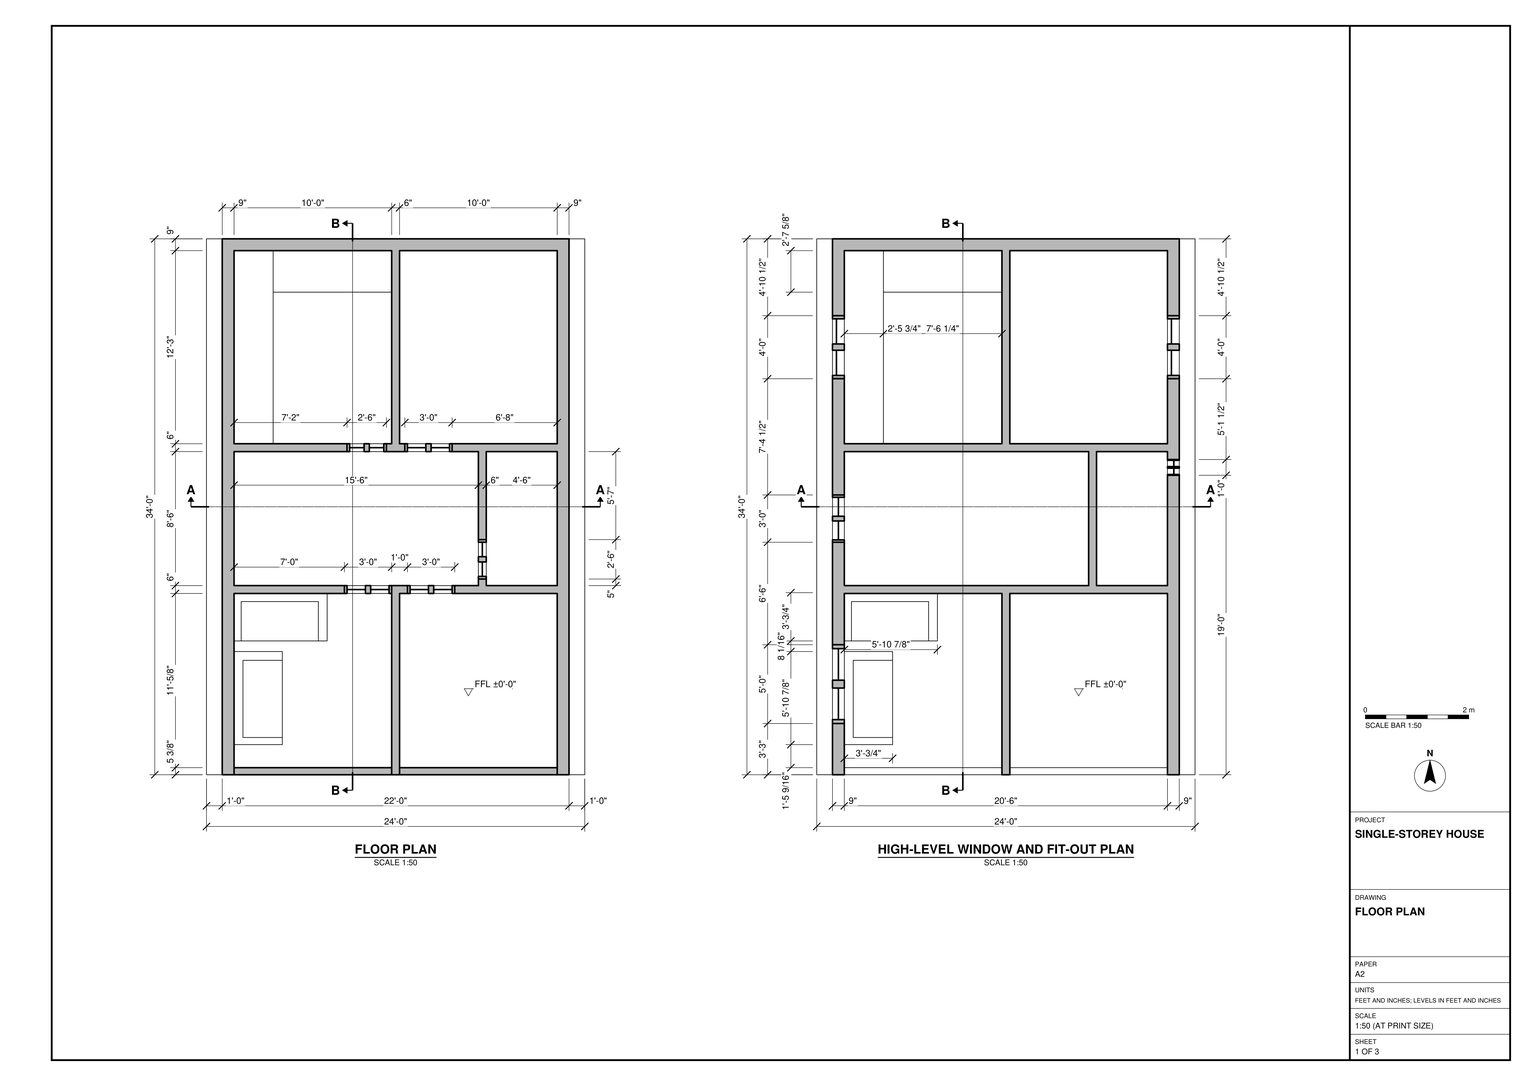
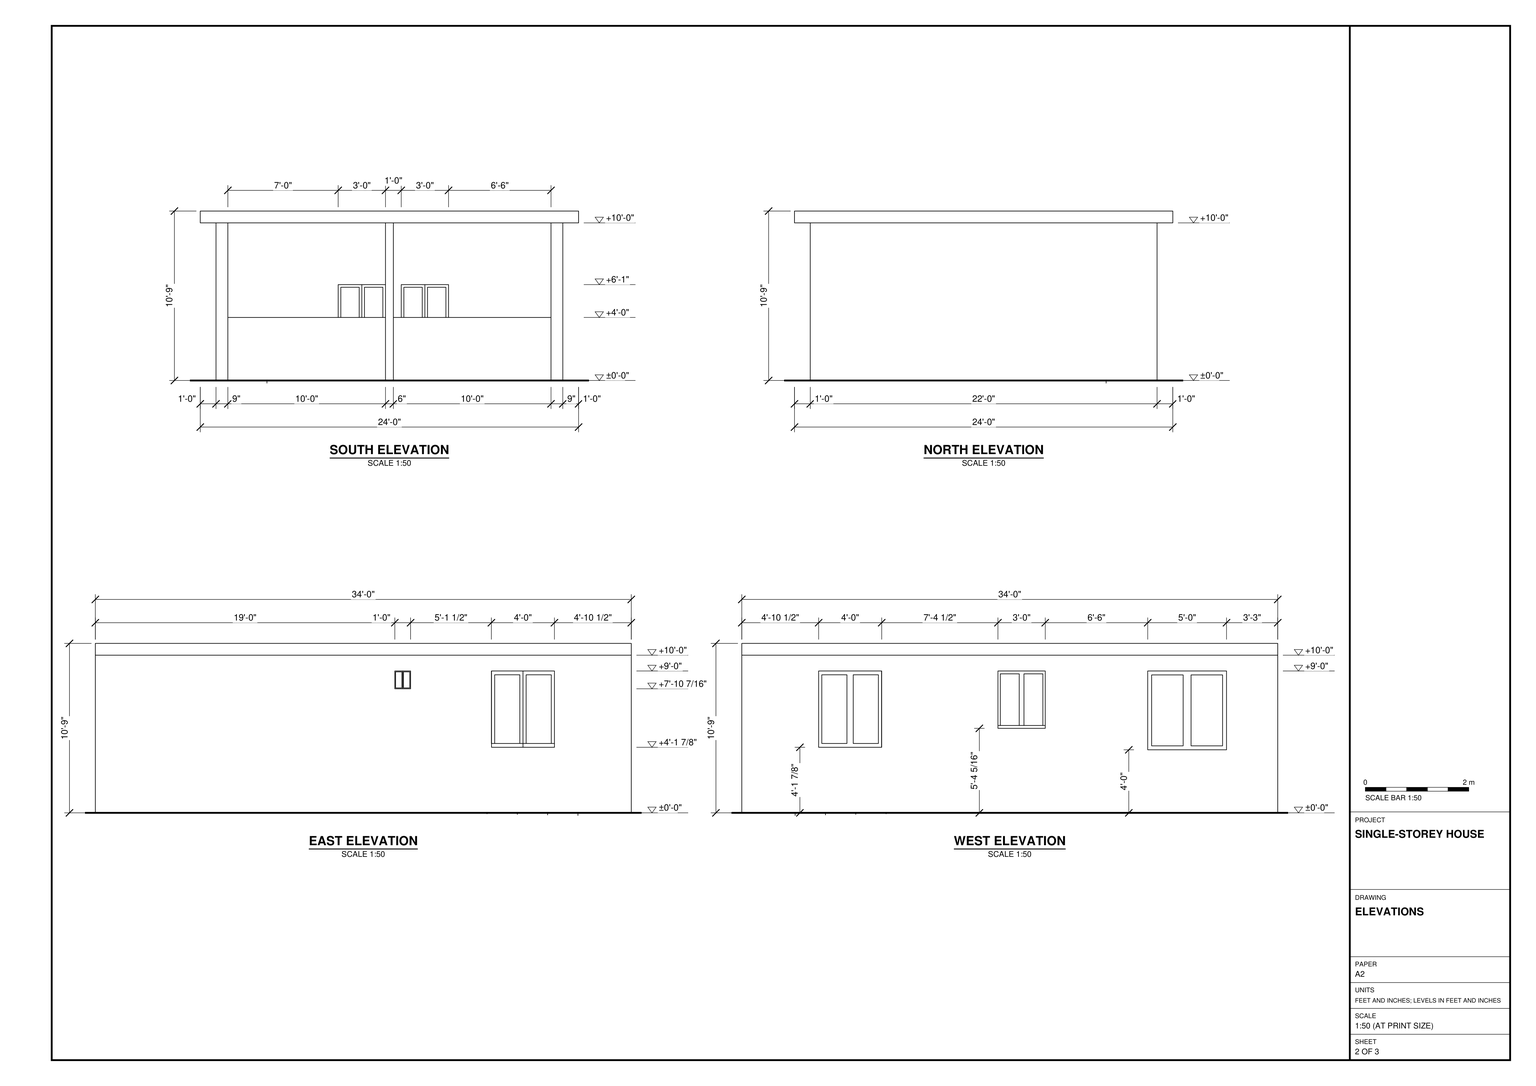
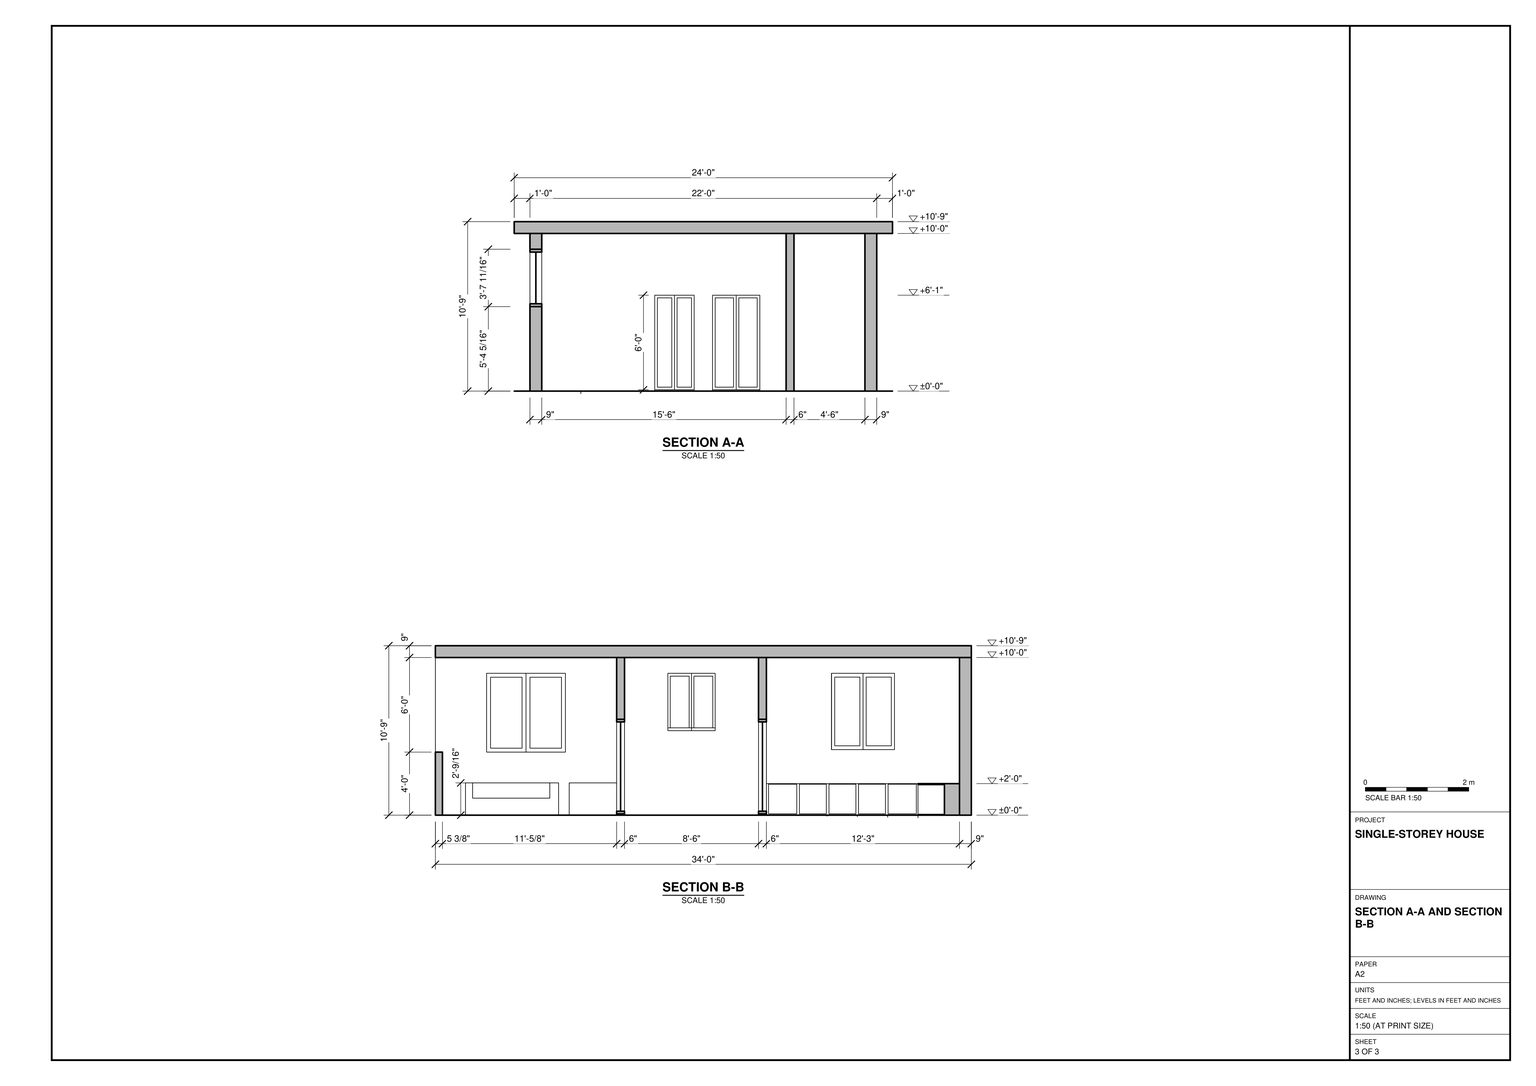
Build the single-storey house shown in task_files/diagram_01.pdf. Work in feet and inches. Set the finished floor at ±0'-0" and orient the plan with north at the top. The overall dimensions, including the roof, are 24'-0" east to west, 34'-0" north to south and 10'-9" high.

Model the floor, the 9" full-height exterior walls and the 6" interior partitions. Divide each end of the house into two equal-width rooms. In the middle band, place the wider room on the west and the narrow room on the east. Use the sections to distinguish the low south wall from the full-height walls behind it. Set the underside of the flat roof at +10'-0" and extend it 1'-0" beyond each side wall.

Use the floor plan to place the interior door units and the high-level plan to locate the exterior windows. Match the window widths and sill heights to the elevations rather than repeating one window size throughout. Model the low built-in joinery in the northwest room and the two low furniture pieces set at right angles in the southwest room. Any decor or loose items may be represented by suitable library components.

Keep the shell elements, including the walls, floor slab and roof, and each furniture or joinery piece in separate groups or components. Use components for repeated parts. Save one SketchUp model as output_files/single_storey_house_with_an_overhanging_flat_roof.skp.

# SketchUp Ruby script. Lengths in inches.
U = 1.inch
M = Sketchup.active_model
def pt(a) = Geom::Point3d.new(a.map { |v| v * U })
def face(e, loops, mat)
  f = e.add_face(loops[0].map { |a| pt(a) })
  loops[1..].each { |l| e.add_face(l.map { |a| pt(a) }).erase! }
  f.material = f.back_material = mat if mat
  f
end
# faces: each face lists its corners as indices into pts; further lists are holes
def faces(e, pts, list, mat = nil) = list.each { |f| face(e, (f[0].is_a?(Array) ? f : [f]).map { |l| l.map { |i| pts[i] } }, mat) }
# xy, xz, yz: faces in a plane at the given z, y or x. An outline is a flat list of corners, or four numbers for a rectangle; further outlines are holes
def ring(l) = l.size == 4 ? [[l[0], l[1]], [l[2], l[1]], [l[2], l[3]], [l[0], l[3]]] : l.each_slice(2).to_a
def flat(e, list, mat, &to3) = list.each { |f| face(e, (f[0].is_a?(Array) ? f : [f]).map { |l| ring(l).map { |u, v| to3.(u, v) } }, mat) }
def xy(e, z, list, mat = nil) = flat(e, list, mat) { |x, y| [x, y, z] }
def xz(e, y, list, mat = nil) = flat(e, list, mat) { |x, z| [x, y, z] }
def yz(e, x, list, mat = nil) = flat(e, list, mat) { |y, z| [x, y, z] }
def lines(e, pts, list) = list.each { |a, b| e.add_line(pt(pts[a]), pt(pts[b])) }
# prism: a flat outline (further loops are holes) pulled along v
def prism(e, loops, v, mat = nil)
  f = face(e, loops, mat); d = Geom::Vector3d.new(v.map { |x| x * U })
  f.pushpull(f.normal.samedirection?(d) ? d.length : -d.length)
end
def box(e, o, s, mat = nil) = prism(e, [[o, [o[0] + s[0], o[1], o[2]], [o[0] + s[0], o[1] + s[1], o[2]], [o[0], o[1] + s[1], o[2]]]], [0, 0, s[2]], mat)
def at(x, y, z, deg = 0) = Geom::Transformation.translation(pt([x, y, z])) * Geom::Transformation.rotation(ORIGIN, Z_AXIS, deg.degrees)
def axes(o, x, y, z) = Geom::Transformation.new([*x, 0, *y, 0, *z, 0, *pt(o).to_a, 1])
def part(name) = M.definitions.add(name)
# library, detail: a bought-in or finely detailed component or shape, given as its bounding box
def library(name, o, s) = part(name).tap { |d| box(d.entities, o, s) }
def detail(e, o, s) = box(e.add_group.entities, o, s)
def put(e, d, t, mat = nil) = e.add_instance(d, t).tap { |i| i.material = mat if mat }
def group(e, t, mat = nil) = e.add_group.tap { |g| g.transformation = t; g.material = mat if mat }.entities
root = M.entities
M.materials.add("[Carrera Marble]").color = [207, 207, 207]
M.materials.add("[Color M06]").color = [86, 86, 86]
M.materials.add("[Fencing Picket Concave]").color = [160, 160, 160]
M.materials.add("[Stone Brushed Khaki]").color = [226, 197, 133]
M.materials.add("[Translucent Glass Blue]").color = [100, 149, 237]
M.materials["[Translucent Glass Blue]"].alpha = 0.5
M.materials.add("[Wood Cherry Original]").color = [152, 86, 42]
M.materials.add("[Wood Floor]").color = [155, 105, 61]
M.materials.add("[Wood OSB]").color = [240, 195, 122]
c1 = part("Component\#1")
xy(c1.entities,0,[[0,0,36.75,70.875]],"[Carrera Marble]")
xy(c1.entities,12.9375,[[6.77,5.43,36.75,64.17]],"[Color M06]")
xy(c1.entities,24.5625,[[0,0,36.75,0,36.75,5.43,6.77,5.43,6.77,64.17,36.75,64.17,36.75,70.875,0,70.875]],"[Color M06]")
xz(c1.entities,0,[[0,0,36.75,24.5625]],"[Color M06]")
xz(c1.entities,5.43,[[6.77,12.9375,36.75,24.5625]],"[Color M06]")
xz(c1.entities,64.17,[[6.77,12.9375,36.75,24.5625]],"[Color M06]")
xz(c1.entities,70.875,[[0,0,36.75,24.5625]],"[Color M06]")
yz(c1.entities,0,[[0,0,70.875,24.5625]],"[Carrera Marble]")
yz(c1.entities,6.77,[[5.43,12.9375,64.17,24.5625]],"[Color M06]")
yz(c1.entities,36.75,[[0,0,70.875,0,70.875,24.5625,64.17,24.5625,64.17,12.9375,5.43,12.9375,5.43,24.5625,0,24.5625]],"[Color M06]")
c2 = part("Group\#2")
xy(c2.entities,0,[[0,0,9,30],[0,30,9,60]])
xy(c2.entities,3,[[0,3,4.5,27],[4.5,3,9,27],[0,33,4.5,57],[4.5,33,9,57]])
xy(c2.entities,57,[[0,3,4.5,27],[4.5,3,9,27],[0,33,4.5,57],[4.5,33,9,57]])
xy(c2.entities,60,[[0,0,9,30],[0,30,9,60]])
xz(c2.entities,0,[[0,0,9,60]])
xz(c2.entities,3,[[0,3,4.5,57],[4.5,3,9,57]])
xz(c2.entities,27,[[0,3,4.5,57],[4.5,3,9,57]])
xz(c2.entities,33,[[0,3,4.5,57],[4.5,3,9,57]])
xz(c2.entities,57,[[0,3,4.5,57],[4.5,3,9,57]])
xz(c2.entities,60,[[0,0,9,60]])
yz(c2.entities,0,[[[0,0,60,60],[3,3,27,57],[33,3,57,57]]])
yz(c2.entities,4.5,[[3,3,27,57],[33,3,57,57]],"[Translucent Glass Blue]")
yz(c2.entities,9,[[[0,0,30,60],[3,3,27,57]],[[30,0,60,60],[33,3,57,57]]])
c3 = part("Group\#5")
xy(c3.entities,0,[[0,0,36,6]],"[Carrera Marble]")
xy(c3.entities,1,[[0,0,36,6]],"[Stone Brushed Khaki]")
xz(c3.entities,0,[[0,0,36,1]],"[Stone Brushed Khaki]")
xz(c3.entities,6,[[0,0,36,1]],"[Stone Brushed Khaki]")
yz(c3.entities,0,[[0,0,6,1]],"[Carrera Marble]")
yz(c3.entities,36,[[0,0,6,1]],"[Carrera Marble]")
c4 = part("Group\#3")
xy(c4.entities,0,[[0,0,30,6]])
xy(c4.entities,1,[[0,0,30,6]],"[Wood OSB]")
xz(c4.entities,0,[[0,0,30,1]],"[Wood OSB]")
xz(c4.entities,6,[[0,0,30,1]],"[Wood OSB]")
yz(c4.entities,0,[[0,0,6,1]])
yz(c4.entities,30,[[0,0,6,1]])
c5 = part("Group\#9")
xy(c5.entities,0,[[0,-6,15,0],[15,-6,30,0]])
xy(c5.entities,2,[[2,-6,13,-3],[17,-6,28,-3],[2,-3,13,0],[17,-3,28,0]])
xy(c5.entities,70,[[2,-6,13,-3],[17,-6,28,-3],[2,-3,13,0],[17,-3,28,0]])
xy(c5.entities,72,[[0,-6,30,0]])
xz(c5.entities,-6,[[[0,0,15,72],[2,2,13,70]],[[15,0,30,72],[17,2,28,70]]])
xz(c5.entities,-3,[[2,2,13,70],[17,2,28,70]])
xz(c5.entities,0,[[[0,0,30,72],[17,2,28,70],[2,2,13,70]]])
yz(c5.entities,0,[[-6,0,0,72]])
yz(c5.entities,2,[[-6,2,-3,70],[-3,2,0,70]])
yz(c5.entities,13,[[-6,2,-3,70],[-3,2,0,70]])
yz(c5.entities,17,[[-6,2,-3,70],[-3,2,0,70]])
yz(c5.entities,28,[[-6,2,-3,70],[-3,2,0,70]])
yz(c5.entities,30,[[-6,0,0,72]])
c6 = part("Group\#11")
xy(c6.entities,0,[[0,0,120,5.39]],"[Carrera Marble]")
xy(c6.entities,48,[[0,0,120,5.39]],"[Carrera Marble]")
xz(c6.entities,0,[[0,0,120,48]],"[Fencing Picket Concave]")
xz(c6.entities,5.39,[[0,0,120,48]],"[Carrera Marble]")
yz(c6.entities,0,[[0,0,5.39,48]],"[Carrera Marble]")
yz(c6.entities,120,[[0,0,5.39,48]],"[Carrera Marble]")
xy(root,0,[[0,0,12,408],[12,0,21,0,21,138,105,138,105,144,21,144,21,246,107,246,107,252,21,252,21,399,141,399,141,252,137,252,137,246,151,246,151,252,147,252,147,399,267,399,267,252,187,252,187,246,207,246,207,179,213,179,213,246,267,246,267,144,213,144,213,149,207,149,207,144,189,144,189,138,267,138,267,0,276,0,276,408,12,408],[276,0,288,408],[107,246,137,252]])
xy(root,0,[[147,0,267,0,267,138,189,138,189,144,207,144,207,149,213,149,213,144,267,144,267,246,213,246,213,179,207,179,207,246,21,246,21,144,153,144,153,138,147,138],[21,5.39,141,138],[50.76,252,141,367.4],[147,252,267,399]],"[Carrera Marble]")
xy(root,48,[[12,39,21,99]])
xy(root,49.9,[[12,301.5,21,349.5]])
xy(root,52.81,[[267,301.5,276,349.5]])
xy(root,66.5,[[12,177,21,213]])
xy(root,73,[[105,138,141,144],[153,138,189,144],[207,149,213,179],[107,246,137,252],[151,246,187,252]])
xy(root,94.43,[[267,228,276,240]])
xy(root,108,[[12,39,21,99],[12,177,21,213],[267,228,276,240],[12,301.5,21,349.5],[267,301.5,276,301.62],
  [267,301.62,276,349.5]])
xy(root,120,[[[12,0,21,0,21,138,141,138,141,0,147,0,147,138,267,138,267,0,276,0,276,408,12,408],[21,144,21,399,141,399,141,252,21,252,21,246,207,246,207,144],[147,252,267,399],[213,144,267,246]]])
xz(root,0,[[12,0,21,120],[141,0,147,120],[267,0,276,120]])
xz(root,39,[[12,48,21,108]])
xz(root,99,[[12,48,21,108]])
xz(root,138,[[21,0,105,0,105,73,141,73,141,120,21,120],[147,0,153,0,153,73,189,73,189,0,267,0,267,120,147,120]])
xz(root,144,[[21,0,21,120,207,120,207,0,189,0,189,73,153,73,153,0,141,0,141,73,105,73,105,0],[213,0,267,120]])
xz(root,149,[[207,0,213,73]])
xz(root,177,[[12,66.5,21,108]])
xz(root,179,[[207,0,213,73]])
xz(root,213,[[12,66.5,21,108]])
xz(root,228,[[267,94.43,276,108]])
xz(root,240,[[267,94.43,276,108]])
xz(root,246,[[21,0,107,0,107,73,137,73,137,0,151,0,151,73,187,73,187,0,207,0,207,120,21,120],[213,0,267,120]])
xz(root,252,[[21,0,21,120,141,120,141,0,137,0,137,73,107,73,107,0],[147,0,147,120,267,120,267,0,187,0,187,73,151,73,151,0]])
xz(root,301.5,[[12,49.9,21,108],[267,52.81,276,108]])
xz(root,349.5,[[12,49.9,21,108],[267,52.81,276,108]])
xz(root,399,[[21,0,141,120],[147,0,267,120]])
xz(root,408,[[12,0,276,120]])
yz(root,12,[[[0,0,408,120],[39,48,99,108],[301.5,49.9,349.5,108],[177,66.5,213,108]]])
yz(root,21,[[[0,0,138,120],[39,48,99,108]],[[144,0,246,120],[177,66.5,213,108]],[[252,0,399,120],[301.5,49.9,349.5,108]]])
yz(root,105,[[138,0,144,73]])
yz(root,107,[[246,0,252,73]])
yz(root,137,[[246,0,252,73]])
yz(root,141,[[0,0,0,120,138,120,138,73,144,73,144,0],[252,0,399,120]])
yz(root,147,[[0,0,138,120],[252,0,399,120]])
yz(root,151,[[246,0,252,73]])
yz(root,153,[[138,0,144,73]])
yz(root,187,[[246,0,252,73]])
yz(root,189,[[138,0,144,73]])
yz(root,207,[[144,0,144,120,246,120,246,0,179,0,179,73,149,73,149,0]])
yz(root,213,[[144,0,149,0,149,73,179,73,179,0,246,0,246,120,144,120]])
yz(root,267,[[0,0,138,120],[[144,0,246,120],[228,94.43,240,108]],[252,0,301.5,120],[301.5,0,349.5,52.81],[349.5,0,349.5,108,301.5,108,301.5,120,399,120,399,0]])
yz(root,276,[[[0,0,408,120],[301.5,52.81,349.5,108],[228,94.43,240,108]]])
p = [[107,246,1],[137,246,1],[50.76,252,24],[50.76,252,0],[50.76,298.16,0],[50.76,298.16,-0.8],
  [50.76,321.24,0],[50.76,321.24,-1.2],[50.76,344.32,0],[50.76,344.32,-1.59],[50.76,367.4,0],[50.76,367.4,-1.99]]
lines(root,p,[[0,1],[2,3],[4,5],[6,7],[8,9],[10,11]])
put(root,c1,at(21,22.93,0),"[Color M06]")
put(root,c1,at(21,138.62,0,-90),"[Color M06]")
put(root,c2,at(12,39,48))
put(root,c2,axes([12,177,64.32],[1,0,0],[0,0.6,0],[0,0,0.72805]))
g1 = group(root,at(9.03,301.62,49.9))
xy(g1,0,[[2.97,0,11.97,23.94],[2.97,23.94,11.97,47.88]])
xy(g1,2.9,[[2.97,2.39,5.99,21.55],[5.99,2.39,11.97,21.55],[2.97,26.33,5.99,45.49],[5.99,26.33,11.97,45.49]])
xy(g1,55.19,[[2.97,2.39,5.99,21.55],[5.99,2.39,11.97,21.55],[2.97,26.33,5.99,45.49],[5.99,26.33,11.97,45.49]])
xy(g1,58.1,[[2.97,0,11.97,23.94],[2.97,23.94,11.97,47.88]])
xz(g1,0,[[2.97,0,11.97,58.1]])
xz(g1,2.39,[[2.97,2.9,5.99,55.19],[5.99,2.9,11.97,55.19]])
xz(g1,21.55,[[2.97,2.9,5.99,55.19],[5.99,2.9,11.97,55.19]])
xz(g1,26.33,[[2.97,2.9,5.99,55.19],[5.99,2.9,11.97,55.19]])
xz(g1,45.49,[[2.97,2.9,5.99,55.19],[5.99,2.9,11.97,55.19]])
xz(g1,47.88,[[2.97,0,11.97,58.1]])
yz(g1,2.97,[[[0,0,47.88,58.1],[2.39,2.9,21.55,55.19],[26.33,2.9,45.49,55.19]]])
yz(g1,5.99,[[2.39,2.9,21.55,55.19],[26.33,2.9,45.49,55.19]],"[Translucent Glass Blue]")
yz(g1,11.97,[[[0,0,23.94,58.1],[2.39,2.9,21.55,55.19]],[[23.94,0,47.88,58.1],[26.33,2.9,45.49,55.19]]])
g2 = group(root,at(264.03,301.62,49.9))
xy(g2,0,[[2.97,0,11.97,23.94],[2.97,23.94,11.97,47.88]])
xy(g2,2.9,[[2.97,2.39,5.98,21.55],[5.98,2.39,11.97,21.55],[2.97,26.33,5.98,45.49],[5.98,26.33,11.97,45.49]])
xy(g2,55.19,[[2.97,2.39,5.98,21.55],[5.98,2.39,11.97,21.55],[2.97,26.33,5.98,45.49],[5.98,26.33,11.97,45.49]])
xy(g2,58.1,[[2.97,0,11.97,23.94],[2.97,23.94,11.97,47.88]])
xz(g2,0,[[2.97,0,11.97,58.1]])
xz(g2,2.39,[[2.97,2.9,5.98,55.19],[5.98,2.9,11.97,55.19]])
xz(g2,21.55,[[2.97,2.9,5.98,55.19],[5.98,2.9,11.97,55.19]])
xz(g2,26.33,[[2.97,2.9,5.98,55.19],[5.98,2.9,11.97,55.19]])
xz(g2,45.49,[[2.97,2.9,5.98,55.19],[5.98,2.9,11.97,55.19]])
xz(g2,47.88,[[2.97,0,11.97,58.1]])
yz(g2,2.97,[[[0,0,47.88,58.1],[26.33,2.9,45.49,55.19],[2.39,2.9,21.55,55.19]]])
yz(g2,5.98,[[2.39,2.9,21.55,55.19],[26.33,2.9,45.49,55.19]],"[Translucent Glass Blue]")
yz(g2,11.97,[[[0,0,23.94,58.1],[2.39,2.9,21.55,55.19]],[[23.94,0,47.88,58.1],[26.33,2.9,45.49,55.19]]])
g3 = group(root,at(273.06,227.99,94.43))
xy(g3,0,[[-6.06,0,2.94,6],[-6.06,6,2.94,12.01]])
xy(g3,0.68,[[-6.06,0.6,-1.22,5.4],[-1.22,0.6,2.94,5.4],[-6.06,6.61,-1.22,11.41],[-1.22,6.61,2.94,11.41]])
xy(g3,12.89,[[-6.06,0.6,-1.22,5.4],[-1.22,0.6,2.94,5.4],[-6.06,6.61,-1.22,11.41],[-1.22,6.61,2.94,11.41]])
xy(g3,13.57,[[-6.06,0,2.94,6],[-6.06,6,2.94,12.01]])
xz(g3,0,[[-6.06,0,2.94,13.57]])
xz(g3,0.6,[[-6.06,0.68,-1.22,12.89],[-1.22,0.68,2.94,12.89]])
xz(g3,5.4,[[-6.06,0.68,-1.22,12.89],[-1.22,0.68,2.94,12.89]])
xz(g3,6.61,[[-6.06,0.68,-1.22,12.89],[-1.22,0.68,2.94,12.89]])
xz(g3,11.41,[[-6.06,0.68,-1.22,12.89],[-1.22,0.68,2.94,12.89]])
xz(g3,12.01,[[-6.06,0,2.94,13.57]])
yz(g3,-6.06,[[[0,0,12.01,13.57],[6.61,0.68,11.41,12.89],[0.6,0.68,5.4,12.89]]])
yz(g3,-1.22,[[0.6,0.68,5.4,12.89],[6.61,0.68,11.41,12.89]],"[Translucent Glass Blue]")
yz(g3,2.94,[[[0,0,6,13.57],[0.6,0.68,5.4,12.89]],[[6,0,12.01,13.57],[6.61,0.68,11.41,12.89]]])
g4 = group(root,at(84.01,102,-27.2),"[Wood Floor]")
xy(g4,28.2,[[66.99,144,84.99,150],[84.99,144,102.99,150]])
xy(g4,30.2,[[68.99,144,82.99,147],[86.99,144,100.99,147],[68.99,147,82.99,150],[86.99,147,100.99,150]])
xy(g4,98.2,[[68.99,144,82.99,147],[86.99,144,100.99,147],[68.99,147,82.99,150],[86.99,147,100.99,150]])
xy(g4,100.2,[[66.99,144,84.99,150],[84.99,144,102.99,150]])
xz(g4,144,[[[66.99,28.2,84.99,100.2],[68.99,30.2,82.99,98.2]],[[84.99,28.2,102.99,100.2],[86.99,30.2,100.99,98.2]]])
xz(g4,147,[[68.99,30.2,82.99,98.2],[86.99,30.2,100.99,98.2]])
xz(g4,150,[[[66.99,28.2,102.99,100.2],[68.99,30.2,82.99,98.2],[86.99,30.2,100.99,98.2]]])
yz(g4,66.99,[[144,28.2,150,100.2]])
yz(g4,68.99,[[144,30.2,147,98.2],[147,30.2,150,98.2]])
yz(g4,82.99,[[144,30.2,147,98.2],[147,30.2,150,98.2]])
yz(g4,86.99,[[144,30.2,147,98.2],[147,30.2,150,98.2]])
yz(g4,100.99,[[144,30.2,147,98.2],[147,30.2,150,98.2]])
yz(g4,102.99,[[144,28.2,150,100.2]])
put(root,c3,at(151,246,0),"[Stone Brushed Khaki]")
put(root,c3,at(153,138,0),"[Stone Brushed Khaki]")
g5 = group(root,at(86.01,-6,-27.2),"[Wood Floor]")
xy(g5,28.2,[[66.99,144,84.99,150],[84.99,144,102.99,150]])
xy(g5,30.2,[[68.99,144,82.99,147],[86.99,144,100.99,147],[68.99,147,82.99,150],[86.99,147,100.99,150]])
xy(g5,98.2,[[68.99,144,82.99,147],[86.99,144,100.99,147],[68.99,147,82.99,150],[86.99,147,100.99,150]])
xy(g5,100.2,[[66.99,144,102.99,150]])
xz(g5,144,[[[66.99,28.2,84.99,100.2],[68.99,30.2,82.99,98.2]],[[84.99,28.2,102.99,100.2],[86.99,30.2,100.99,98.2]]])
xz(g5,147,[[68.99,30.2,82.99,98.2],[86.99,30.2,100.99,98.2]])
xz(g5,150,[[[66.99,28.2,102.99,100.2],[68.99,30.2,82.99,98.2],[86.99,30.2,100.99,98.2]]])
yz(g5,66.99,[[144,28.2,150,100.2]])
yz(g5,68.99,[[144,30.2,147,98.2],[147,30.2,150,98.2]])
yz(g5,82.99,[[144,30.2,147,98.2],[147,30.2,150,98.2]])
yz(g5,86.99,[[144,30.2,147,98.2],[147,30.2,150,98.2]])
yz(g5,100.99,[[144,30.2,147,98.2],[147,30.2,150,98.2]])
yz(g5,102.99,[[144,28.2,150,100.2]])
g6 = group(root,at(105,138,0))
box(g6,[0,0,0],[36,6,1],"[Stone Brushed Khaki]")
g7 = group(root,at(38.01,-6,-27.2),"[Wood Floor]")
xy(g7,28.2,[[66.99,144,84.99,150],[84.99,144,102.99,150]])
xy(g7,30.2,[[68.99,144,82.99,147],[86.99,144,100.99,147],[68.99,147,82.99,150],[86.99,147,100.99,150]])
xy(g7,98.2,[[68.99,144,82.99,147],[86.99,144,100.99,147],[68.99,147,82.99,150],[86.99,147,100.99,150]])
xy(g7,100.2,[[66.99,144,84.99,150],[84.99,144,102.99,150]])
xz(g7,144,[[[66.99,28.2,84.99,100.2],[68.99,30.2,82.99,98.2]],[[84.99,28.2,102.99,100.2],[86.99,30.2,100.99,98.2]]])
xz(g7,147,[[68.99,30.2,82.99,98.2],[86.99,30.2,100.99,98.2]])
xz(g7,150,[[[66.99,28.2,102.99,100.2],[86.99,30.2,100.99,98.2],[68.99,30.2,82.99,98.2]]])
yz(g7,66.99,[[144,28.2,150,100.2]])
yz(g7,68.99,[[144,30.2,147,98.2],[147,30.2,150,98.2]])
yz(g7,82.99,[[144,30.2,147,98.2],[147,30.2,150,98.2]])
yz(g7,86.99,[[144,30.2,147,98.2],[147,30.2,150,98.2]])
yz(g7,100.99,[[144,30.2,147,98.2],[147,30.2,150,98.2]])
yz(g7,102.99,[[144,28.2,150,100.2]])
put(root,c4,at(107,246,0))
put(root,c5,at(213,179,1,-90),"[Wood Cherry Original]")
put(root,c4,at(213,149,0,90))
put(root,c5,at(107,252,1),"[Wood Cherry Original]")
put(root,c6,at(21,0,0),"[Fencing Picket Concave]")
put(root,c6,at(147,0,0),"[Fencing Picket Concave]")
g8 = group(root,at(21,252,0))
xy(g8,0,[[0,0,29.76,147]],"[Carrera Marble]")
xy(g8,1.01,[[9.64,1.63,29.76,23.13],[9.64,25.13,29.76,45.63],[9.64,47.63,29.76,68.13],[9.64,70.13,29.76,90.63],[9.64,92.63,29.76,114.13]],"[Carrera Marble]")
xy(g8,23.57,[[9.64,1.63,29.76,23.13],[9.64,25.13,29.76,45.63],[9.64,47.63,29.76,68.13],[9.64,70.13,29.76,90.63],[9.64,92.63,29.76,114.13]],"[Carrera Marble]")
xy(g8,24,[[0,0,29.76,147]],"[Carrera Marble]")
xz(g8,0,[[0,0,29.76,24]],"[Carrera Marble]")
xz(g8,1.63,[[9.64,1.01,29.76,23.57]],"[Carrera Marble]")
xz(g8,23.13,[[9.64,1.01,29.76,23.57]],"[Carrera Marble]")
xz(g8,25.13,[[9.64,1.01,29.76,23.57]],"[Carrera Marble]")
xz(g8,45.63,[[9.64,1.01,29.76,23.57]],"[Carrera Marble]")
xz(g8,47.63,[[9.64,1.01,29.76,23.57]],"[Carrera Marble]")
xz(g8,68.13,[[9.64,1.01,29.76,23.57]],"[Carrera Marble]")
xz(g8,70.13,[[9.64,1.01,29.76,23.57]],"[Carrera Marble]")
xz(g8,90.63,[[9.64,1.01,29.76,23.57]],"[Carrera Marble]")
xz(g8,92.63,[[9.64,1.01,29.76,23.57]],"[Carrera Marble]")
xz(g8,114.13,[[9.64,1.01,29.76,23.57]],"[Carrera Marble]")
xz(g8,147,[[0,0,29.76,24]],"[Carrera Marble]")
yz(g8,0,[[0,0,147,24]],"[Carrera Marble]")
yz(g8,9.64,[[1.63,1.01,23.13,23.57],[25.13,1.01,45.63,23.57],[47.63,1.01,68.13,23.57],[70.13,1.01,90.63,23.57],[92.63,1.01,114.13,23.57]],"[Carrera Marble]")
yz(g8,29.76,[[[0,0,147,0,147,24,1.63,24,1.63,23.57,23.13,23.57,23.13,1.01,1.63,1.01,1.63,24,0,24],[92.63,1.01,114.13,23.57],[70.13,1.01,90.63,23.57],[47.63,1.01,68.13,23.57],[25.13,1.01,45.63,23.57]]],"[Carrera Marble]")
g9 = group(root,at(50.76,367.4,0))
xy(g9,0,[[0,0,90.24,31.6]],"[Carrera Marble]")
xy(g9,0.4375,[[0.3125,0,17.22,20.125],[19.22,0,35.88,20.125],[36.32,0,53.67,20.125],[54.42,0,71.76,20.125],[72.2,0,89.86,20.125]],"[Carrera Marble]")
xy(g9,23.3,[[0.3125,0,17.22,20.125],[19.22,0,35.88,20.125],[36.32,0,53.67,20.125],[54.42,0,71.76,20.125],[72.2,0,89.86,20.125]],"[Carrera Marble]")
xy(g9,24,[[0,0,90.24,31.6]],"[Carrera Marble]")
xz(g9,0,[[[0,0,90.24,24],[19.22,0.4375,19.22,23.3,53.67,23.3,53.67,0.4375,36.32,0.4375,36.32,23.3,35.88,23.3,35.88,0.4375],[72.2,0.4375,89.86,23.3],[54.42,0.4375,71.76,23.3],[0.3125,0.4375,17.22,23.3]]],"[Carrera Marble]")
xz(g9,20.125,[[0.3125,0.4375,17.22,23.3],[19.22,0.4375,35.88,23.3],[36.32,0.4375,53.67,23.3],[54.42,0.4375,71.76,23.3],[72.2,0.4375,89.86,23.3]],"[Carrera Marble]")
xz(g9,31.6,[[0,0,90.24,24]],"[Carrera Marble]")
yz(g9,0,[[0,0,31.6,24]],"[Carrera Marble]")
yz(g9,0.3125,[[0,0.4375,20.125,23.3]],"[Carrera Marble]")
yz(g9,17.22,[[0,0.4375,20.125,23.3]],"[Carrera Marble]")
yz(g9,19.22,[[0,0.4375,20.125,23.3]],"[Carrera Marble]")
yz(g9,35.88,[[0,0.4375,20.125,23.3]],"[Carrera Marble]")
yz(g9,36.32,[[0,0.4375,20.125,23.3]],"[Carrera Marble]")
yz(g9,53.67,[[0,0.4375,20.125,23.3]],"[Carrera Marble]")
yz(g9,54.42,[[0,0.4375,20.125,23.3]],"[Carrera Marble]")
yz(g9,71.76,[[0,0.4375,20.125,23.3]],"[Carrera Marble]")
yz(g9,72.2,[[0,0.4375,20.125,23.3]],"[Carrera Marble]")
yz(g9,89.86,[[0,0.4375,20.125,23.3]],"[Carrera Marble]")
yz(g9,90.24,[[0,0,31.6,24]],"[Carrera Marble]")
g10 = group(root,at(0,0,120))
box(g10,[0,0,0],[288,408,9])
